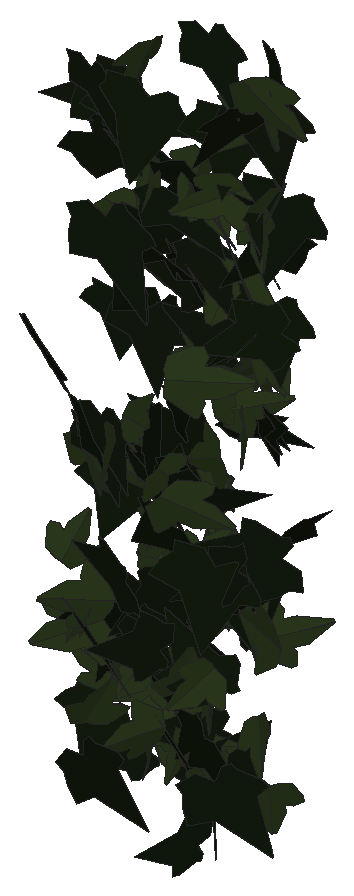
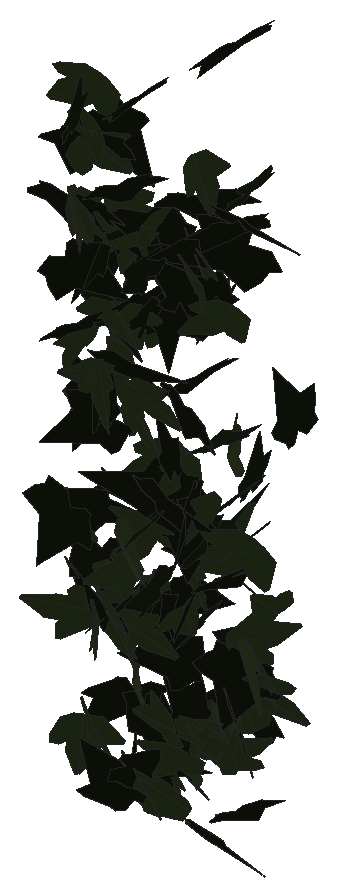
# SketchUp Ruby script. Lengths in inches.
U = 1.inch
M = Sketchup.active_model
def pt(a) = Geom::Point3d.new(a.map { |v| v * U })
def face(e, loops, mat)
  f = e.add_face(loops[0].map { |a| pt(a) })
  loops[1..].each { |l| e.add_face(l.map { |a| pt(a) }).erase! }
  f.material = f.back_material = mat if mat
  f
end
# faces: each face lists its corners as indices into pts; further lists are holes
def faces(e, pts, list, mat = nil) = list.each { |f| face(e, (f[0].is_a?(Array) ? f : [f]).map { |l| l.map { |i| pts[i] } }, mat) }
# xy, xz, yz: faces in a plane at the given z, y or x. An outline is a flat list of corners, or four numbers for a rectangle; further outlines are holes
def ring(l) = l.size == 4 ? [[l[0], l[1]], [l[2], l[1]], [l[2], l[3]], [l[0], l[3]]] : l.each_slice(2).to_a
def flat(e, list, mat, &to3) = list.each { |f| face(e, (f[0].is_a?(Array) ? f : [f]).map { |l| ring(l).map { |u, v| to3.(u, v) } }, mat) }
def xy(e, z, list, mat = nil) = flat(e, list, mat) { |x, y| [x, y, z] }
def xz(e, y, list, mat = nil) = flat(e, list, mat) { |x, z| [x, y, z] }
def yz(e, x, list, mat = nil) = flat(e, list, mat) { |y, z| [x, y, z] }
def lines(e, pts, list) = list.each { |a, b| e.add_line(pt(pts[a]), pt(pts[b])) }
# prism: a flat outline (further loops are holes) pulled along v
def prism(e, loops, v, mat = nil)
  f = face(e, loops, mat); d = Geom::Vector3d.new(v.map { |x| x * U })
  f.pushpull(f.normal.samedirection?(d) ? d.length : -d.length)
end
def box(e, o, s, mat = nil) = prism(e, [[o, [o[0] + s[0], o[1], o[2]], [o[0] + s[0], o[1] + s[1], o[2]], [o[0], o[1] + s[1], o[2]]]], [0, 0, s[2]], mat)
def at(x, y, z, deg = 0) = Geom::Transformation.translation(pt([x, y, z])) * Geom::Transformation.rotation(ORIGIN, Z_AXIS, deg.degrees)
def axes(o, x, y, z) = Geom::Transformation.new([*x, 0, *y, 0, *z, 0, *pt(o).to_a, 1])
def part(name) = M.definitions.add(name)
# library, detail: a bought-in or finely detailed component or shape, given as its bounding box
def library(name, o, s) = part(name).tap { |d| box(d.entities, o, s) }
def detail(e, o, s) = box(e.add_group.entities, o, s)
def put(e, d, t, mat = nil) = e.add_instance(d, t).tap { |i| i.material = mat if mat }
def group(e, t, mat = nil) = e.add_group.tap { |g| g.transformation = t; g.material = mat if mat }.entities
root = M.entities
M.materials.add("1026 AP 7946 SUNNY SIDE UP").color = [254, 231, 186]
M.materials.add("efeu1").color = [18, 25, 13]
M.materials.add("efeu2").color = [43, 57, 29]
c1 = part("ivyleaf_9")
p = [[1.54,2.16,1.25],[1.36,2.04,1.19],[-0.21,0.99,0.68],[-0.71,1.11,0.82],[-0.85,0.86,0.67],[-0.8,0.17,0.21],
  [-0.9,-0.01,0.1],[-0.67,-0.16,-0.02],[-0.08,-0.08,-0.05],[-0.03,-0.6,-0.4],[0.65,-0.88,-0.66],[0.83,-0.6,-0.49],
  [1.29,-0.42,-0.43],[1.8125,-0.07,-0.26],[1.21,0.44,0.15]]
faces(c1.entities,p,[[0,1,2,3,4,5,6,7,8,9,10,11,12,13,14]],"efeu1")
c2 = part("ivyleaf_10")
p = [[0,0.5,-0.03],[-0.0625,2.02,-0.43],[-0.19,2.01,-0.46],[-0.54,1.05,-0.29],[-0.52,0.625,-0.18],[-0.83,0.76,-0.28],
  [-1.16,0.64,-0.33],[-1.15,0.33,-0.24],[-0.77,-0.39,0.02],[-0.3,-0.51,0.16],[0.04,-0.48,0.23],[-0.02,2.01,-0.4375],
  [-0.06,2.01,-0.43],[0.04,-0.49,0.23],[0.67,-0.49,0.14],[1.38,0.36,-0.2],[1.375,0.51,-0.24],[0.81,0.65,-0.19],
  [0.62,0.59,-0.15],[0.6,1.09,-0.28],[0.5,1.23,-0.31]]
faces(c2.entities,p,[[0,1,2,3,4,5,6,7,8,9,10],[11,12,0,13,14,15,16,17,18,19,20]],"efeu2")
put(root,c1,axes([127.27,207.86,278.51],[0.09991,-0.42403,-0.09348],[-0.00995,0.08836,-0.44114],[0.68098,0.0635,0.00727]),"1026 AP 7946 SUNNY SIDE UP")
put(root,c1,axes([126.99,209.29,271.18],[-0.37733,0.18301,0.11018],[-0.15539,0.04456,-0.30973],[-0.29394,-0.25849,0.0223]),"1026 AP 7946 SUNNY SIDE UP")
put(root,c1,axes([125.64,209.45,268.95],[-0.00188,-0.09667,-0.35246],[0.53425,0.09867,-0.02942],[0.16176,-0.32702,0.09306]),"1026 AP 7946 SUNNY SIDE UP")
put(root,c1,axes([125.98,209.8125,271.66],[0.16936,-0.34122,-0.00918],[0.03095,-0.00109,0.36812],[-0.53575,-0.10793,0.01836]),"1026 AP 7946 SUNNY SIDE UP")
put(root,c1,axes([127.4,210,272.25],[-0.29374,-0.33207,-0.04474],[0.06069,0.02588,-0.39177],[0.5227,-0.18962,0.02034]),"1026 AP 7946 SUNNY SIDE UP")
put(root,c1,axes([127.26,209.77,268.05],[-0.34107,0.22543,0.04372],[-0.06924,0.01462,-0.32145],[-0.35361,-0.2203,0.02077]),"1026 AP 7946 SUNNY SIDE UP")
put(root,c2,axes([125.53,210.08,273.42],[0.03461,-0.00665,0.3661],[0.31545,-0.29372,-0.02018],[0.46141,0.20131,-0.01366]),"1026 AP 7946 SUNNY SIDE UP")
put(root,c2,axes([127.24,210.04,270.52],[0.16585,0.14434,-0.27042],[-0.20229,-0.23045,-0.18458],[-0.42663,0.16538,-0.01761]),"1026 AP 7946 SUNNY SIDE UP")
put(root,c2,axes([126.84,210.03,270.27],[-0.20114,-0.2859,-0.02326],[-0.0199,-0.01729,0.32254],[-0.45032,0.12847,-0.00387]),"1026 AP 7946 SUNNY SIDE UP")
put(root,c1,axes([125.02,210.1875,270.45],[0.25152,-0.2589,0.1894],[0.11164,-0.17317,-0.31337],[0.48804,0.17304,-0.02593]),"1026 AP 7946 SUNNY SIDE UP")
put(root,c1,axes([124.21,210.29,274.39],[0.02602,-0.13736,0.34062],[0.15547,-0.31717,-0.14236],[0.54225,0.09753,0.02447]),"1026 AP 7946 SUNNY SIDE UP")
put(root,c1,axes([126.1,210.04,270.95],[0.15449,-0.22762,-0.19575],[-0.12607,0.17091,-0.25436],[0.44751,0.12673,-0.00408]),"1026 AP 7946 SUNNY SIDE UP")
put(root,c2,axes([126.93,209.9,275.06],[0.05772,-0.07931,-0.37891],[0.47007,0.22983,-0.019],[0.3581,-0.28892,0.08601]),"1026 AP 7946 SUNNY SIDE UP")
put(root,c1,axes([127.65,210.14,272.23],[-0.43689,0.15575,-0.01515],[0.00086,-0.03079,-0.32718],[-0.24612,-0.27657,0.02575]),"1026 AP 7946 SUNNY SIDE UP")
put(root,c2,axes([125.21,210.12,269.19],[-0.17822,-0.27692,0.07402],[0.03531,0.07013,0.30861],[-0.4491,0.11541,-0.00511]),"1026 AP 7946 SUNNY SIDE UP")
put(root,c1,axes([127.4,210.08,268.9],[-0.01795,-0.22714,-0.28826],[0.05185,0.27683,-0.23235],[0.56274,-0.03275,0.01221]),"1026 AP 7946 SUNNY SIDE UP")
put(root,c1,axes([126.53,210.125,272.57],[0.14554,0.01847,-0.30587],[-0.45919,-0.05415,-0.09754],[-0.08995,0.30634,0.00305]),"1026 AP 7946 SUNNY SIDE UP")
put(root,c1,axes([124.9,210.47,273.28],[-0.0612,-0.09787,0.31696],[-0.00972,-0.31016,-0.10408],[0.5084,-0.01771,0.03616]),"1026 AP 7946 SUNNY SIDE UP")
put(root,c1,axes([127.17,210.23,270.29],[-0.39411,-0.2107,0.0742],[0.06415,0.06497,0.33687],[-0.34482,0.2529,-0.02213]),"1026 AP 7946 SUNNY SIDE UP")
put(root,c2,axes([126.62,210.11,272.98],[-0.24055,-0.14641,-0.30892],[0.38349,0.17475,-0.21566],[0.3564,-0.28686,0.02355]),"1026 AP 7946 SUNNY SIDE UP")
put(root,c2,axes([124.96,210.54,270.7],[0.00384,0.10084,0.37452],[-0.09963,-0.3577,0.10072],[0.58391,-0.0617,0.01472]),"1026 AP 7946 SUNNY SIDE UP")
put(root,c2,axes([125.82,210.59,268.97],[0.00712,-0.02337,0.36221],[-0.00975,-0.3517,-0.02605],[0.55418,-0.00589,-0.00512]),"1026 AP 7946 SUNNY SIDE UP")
put(root,c1,axes([125.49,210.66,275.79],[-0.06401,-0.17767,0.34495],[-0.0686,-0.33335,-0.18907],[0.59349,-0.05769,0.01535]),"1026 AP 7946 SUNNY SIDE UP")
put(root,c1,axes([126.07,210.77,271.18],[-0.01476,-0.05724,-0.38375],[0.18924,-0.35322,0.05077],[-0.56104,-0.11764,0.02722]),"1026 AP 7946 SUNNY SIDE UP")
put(root,c2,axes([126.57,210.73,268.27],[-0.00143,-0.11934,0.32477],[0.28541,-0.26659,-0.10476],[0.44781,0.16953,0.06781]),"1026 AP 7946 SUNNY SIDE UP")
put(root,c2,axes([127.12,210.4,273.7],[-0.20162,0.12835,0.2681],[-0.40277,0.082,-0.17168],[-0.21219,-0.27761,0.07113]),"1026 AP 7946 SUNNY SIDE UP")
put(root,c2,axes([126.2,210.4,273.15],[-0.10446,-0.21988,-0.21946],[0.16823,0.18622,-0.23266],[0.44958,-0.12077,0.03607]),"1026 AP 7946 SUNNY SIDE UP")
put(root,c2,axes([124.68,210.57,270.49],[0.28346,-0.25845,-0.03715],[-0.04145,0.02377,-0.32438],[0.40792,0.18201,-0.00715]),"1026 AP 7946 SUNNY SIDE UP")
put(root,c2,axes([124.68,210.68,270.14],[0.36279,0.00726,-0.25397],[-0.38216,-0.05104,-0.23614],[-0.06633,0.3338,-0.02858]),"1026 AP 7946 SUNNY SIDE UP")
put(root,c1,axes([126.74,210.8,268.31],[-0.03358,-0.01568,-0.35261],[0.4759,-0.16144,-0.01278],[-0.25226,-0.30247,0.02283]),"1026 AP 7946 SUNNY SIDE UP")
put(root,c2,axes([127.26,210.37,274.67],[0.02198,0.06976,0.31894],[-0.10522,0.30317,-0.06557],[-0.48717,-0.06233,0.02855]),"1026 AP 7946 SUNNY SIDE UP")
put(root,c1,axes([127.9,210.72,275.73],[-0.46783,0.00402,0.10863],[-0.16563,-0.02873,-0.30531],[0.00915,-0.31434,0.02744]),"1026 AP 7946 SUNNY SIDE UP")
put(root,c2,axes([125.625,210.82,268.53],[-0.05408,0.05838,0.32312],[0.30635,-0.24555,0.06773],[0.3966,0.19763,-0.00826]),"1026 AP 7946 SUNNY SIDE UP")
put(root,c2,axes([124.5,210.43,271.34],[0.13703,0.18573,-0.23167],[0.12732,0.21121,0.21229],[0.44192,-0.11845,0.01068]),"1026 AP 7946 SUNNY SIDE UP")
put(root,c1,axes([126.02,210.88,268.625],[-0.07889,-0.08642,0.34051],[0.11879,-0.3291,-0.07864],[0.52467,0.06152,0.06901]),"1026 AP 7946 SUNNY SIDE UP")
put(root,c1,axes([126.95,210.9,276.65],[0.2821,-0.17295,-0.30518],[0.44193,-0.11567,0.24506],[-0.30689,-0.32555,0.07237]),"1026 AP 7946 SUNNY SIDE UP")
put(root,c2,axes([127.98,210.45,271.16],[0.04232,-0.07884,-0.38868],[-0.34476,0.30738,-0.08058],[0.49762,0.21966,-0.02277]),"1026 AP 7946 SUNNY SIDE UP")
put(root,c2,axes([124.93,210.51,272.82],[-0.14254,0.25438,0.15434],[-0.09747,0.13528,-0.27717],[-0.45268,-0.10923,0.01108]),"1026 AP 7946 SUNNY SIDE UP")
put(root,c1,axes([124.81,210.83,273.3],[0.10859,-0.32056,0.01121],[-0.00415,-0.01356,-0.33785],[0.50442,0.06889,-0.00519]),"1026 AP 7946 SUNNY SIDE UP")
put(root,c1,axes([127.79,210.87,272.17],[-0.14084,-0.14988,-0.31774],[-0.32064,-0.23192,0.17624],[-0.432,0.22099,-0.02722]),"1026 AP 7946 SUNNY SIDE UP")
put(root,c1,axes([126.26,210.5625,272.63],[0.14978,0.04082,0.33982],[0.51087,0.05978,-0.104],[-0.10848,0.33787,-0.02059]),"1026 AP 7946 SUNNY SIDE UP")
put(root,c1,axes([126.69,210.65,269.11],[0.20222,-0.02875,-0.33271],[-0.50958,-0.01195,-0.13199],[-0.0008,0.34727,-0.03004]),"1026 AP 7946 SUNNY SIDE UP")
put(root,c1,axes([127.47,210.74,275.58],[-0.26572,0.25247,-0.09249],[0.06154,-0.08346,-0.31317],[-0.41759,-0.17295,0.0127]),"1026 AP 7946 SUNNY SIDE UP")
put(root,c2,axes([126.55,210.99,269.73],[0.11557,-0.11452,0.32943],[0.32122,-0.24731,-0.14078],[0.4279,0.21659,0.01671]),"1026 AP 7946 SUNNY SIDE UP")
put(root,c2,axes([126.67,210.55,271.79],[0.14921,0.14974,-0.31156],[0.18275,0.28137,0.18223],[0.49945,-0.14769,0.0264]),"1026 AP 7946 SUNNY SIDE UP")
put(root,c2,axes([127.14,211.03,274.13],[0.15521,-0.20932,0.29815],[0.28379,-0.23129,-0.23614],[0.48641,0.20174,0.04263]),"1026 AP 7946 SUNNY SIDE UP")
put(root,c1,axes([125.51,210.82,270.98],[0.26552,-0.27145,-0.12209],[-0.08652,0.10349,-0.32865],[0.45665,0.17744,0.00872]),"1026 AP 7946 SUNNY SIDE UP")
put(root,c1,axes([125.39,210.94,275.99],[0.1155,-0.09534,0.29048],[0.28402,-0.21726,-0.12519],[0.37301,0.19495,0.00538]),"1026 AP 7946 SUNNY SIDE UP")
put(root,c1,axes([124.83,210.68,270.42],[0.33032,0.24724,-0.03375],[-0.01325,-0.0376,-0.33395],[-0.39224,0.20948,-0.01714]),"1026 AP 7946 SUNNY SIDE UP")
put(root,c1,axes([125.45,211.03,275.09],[-0.03538,-0.37488,0.0251],[0.00109,-0.02658,-0.38704],[0.59093,-0.02239,0.00222]),"1026 AP 7946 SUNNY SIDE UP")
put(root,c2,axes([127.67,210.84,268.53],[-0.33662,-0.25238,-0.03652],[0.05863,0.0129,-0.34024],[0.39612,-0.21638,0.01932]),"1026 AP 7946 SUNNY SIDE UP")
put(root,c1,axes([125.51,211.04,269.52],[0.05115,-0.0848,0.32343],[0.19244,-0.28965,-0.09521],[0.47454,0.1266,0.00375]),"1026 AP 7946 SUNNY SIDE UP")
put(root,c2,axes([127.26,210.65,274.41],[0.04171,-0.0045,-0.34676],[0.34711,0.2551,0.0159],[0.39954,-0.22115,0.02238]),"1026 AP 7946 SUNNY SIDE UP")
put(root,c1,axes([124.47,211.03,278.45],[0.11901,-0.30664,0.06791],[0.03001,-0.06498,-0.32574],[0.49284,0.078,0.00344]),"1026 AP 7946 SUNNY SIDE UP")
put(root,c2,axes([125.86,210.86,271.97],[0.35971,-0.22556,-0.15011],[-0.16316,0.10047,-0.33037],[0.38825,0.2512,0.00023]),"1026 AP 7946 SUNNY SIDE UP")
put(root,c2,axes([126.85,211.05,277.375],[0.22311,0.08163,-0.30419],[-0.38043,-0.17057,-0.16909],[-0.29662,0.28017,-0.01193]),"1026 AP 7946 SUNNY SIDE UP")
put(root,c1,axes([127.32,210.81,271.49],[-0.0268,0.34631,-0.09795],[-0.00633,-0.09734,-0.35766],[-0.56548,-0.01532,0.00864]),"1026 AP 7946 SUNNY SIDE UP")
put(root,c1,axes([127.07,210.97,278.6875],[-0.06803,0.25081,-0.24763],[0.06298,-0.23846,-0.2636],[-0.54418,-0.05896,0.00045]),"1026 AP 7946 SUNNY SIDE UP")
put(root,c2,axes([127.36,210.96,279.17],[-0.3807,-0.00009,-0.24392],[0.36636,-0.06033,-0.24578],[-0.06622,-0.33323,0.04255]),"1026 AP 7946 SUNNY SIDE UP")
put(root,c1,axes([126.39,210.86,270.77],[0.10181,-0.09867,0.27903],[-0.1404,0.25768,0.11995],[-0.43185,-0.10704,0.02678]),"1026 AP 7946 SUNNY SIDE UP")
put(root,c2,axes([125.99,211.04,268.63],[0.32056,-0.20487,0.05146],[0.03358,-0.05068,-0.29731],[0.33031,0.20397,-0.01971]),"1026 AP 7946 SUNNY SIDE UP")
put(root,c2,axes([127.04,210.73,274.58],[0.06583,-0.04009,0.32051],[-0.05262,0.31174,0.04781],[-0.49078,-0.0388,0.03787]),"1026 AP 7946 SUNNY SIDE UP")
put(root,c1,axes([126.26,211.2,275.73],[-0.09104,0.0095,0.33014],[-0.34085,-0.24102,-0.0344],[0.37132,-0.21892,0.04937]),"1026 AP 7946 SUNNY SIDE UP")
put(root,c1,axes([125.42,210.92,276.26],[-0.10622,-0.03832,0.30642],[0.47125,0.00731,0.07108],[-0.02463,0.30513,0.03859]),"1026 AP 7946 SUNNY SIDE UP")
put(root,c2,axes([127.21,211.15,277.03],[0.31563,-0.09633,0.22963],[0.2801,-0.13914,-0.22747],[0.26063,0.26619,-0.03361]),"1026 AP 7946 SUNNY SIDE UP")
put(root,c1,axes([127.09,211.21,274.01],[-0.00037,-0.07222,0.35978],[0.21834,-0.32214,-0.07034],[0.5172,0.13594,0.02995]),"1026 AP 7946 SUNNY SIDE UP")
put(root,c2,axes([125.36,211.13,277.23],[0.35508,-0.17658,0.11695],[0.11653,-0.09051,-0.29482],[0.30974,0.23647,-0.02316]),"1026 AP 7946 SUNNY SIDE UP")
put(root,c1,axes([125.77,211.18,273.59],[-0.01857,0.03451,0.30122],[0.08363,-0.28736,0.0355],[0.45502,0.05422,0.00577]),"1026 AP 7946 SUNNY SIDE UP")
put(root,c2,axes([124.57,211.01,270.83],[0.1814,-0.33764,-0.12243],[-0.08,0.10609,-0.3667],[0.55611,0.1254,-0.01282]),"1026 AP 7946 SUNNY SIDE UP")
put(root,c1,axes([125.25,211.23,278.19],[-0.31977,-0.3193,-0.04958],[0.06651,0.02789,-0.38925],[0.50294,-0.2067,0.01995]),"1026 AP 7946 SUNNY SIDE UP")
put(root,c1,axes([124.45,211.2,272.82],[0.07282,-0.32278,0.02636],[-0.00106,-0.0278,-0.33606],[0.50937,0.04608,-0.00447]),"1026 AP 7946 SUNNY SIDE UP")
put(root,c1,axes([125.875,211.08,277.17],[0.19198,-0.05348,0.29158],[0.41463,-0.10377,-0.13785],[0.18343,0.29055,0.00641]),"1026 AP 7946 SUNNY SIDE UP")
put(root,c2,axes([124.8125,211.15,269.19],[0.20131,0.17687,0.21535],[-0.23465,-0.1471,0.22258],[0.35957,-0.19501,0.02469]),"1026 AP 7946 SUNNY SIDE UP")
put(root,c2,axes([126.07,211.32,277.42],[-0.10076,-0.16907,0.29259],[0.18064,-0.28358,-0.14837],[0.4887,0.06996,0.11517]),"1026 AP 7946 SUNNY SIDE UP")
put(root,c1,axes([125.16,211.2,272.62],[0.28068,-0.2741,0.0578],[0.02707,-0.05751,-0.33687],[0.43959,0.17855,-0.01616]),"1026 AP 7946 SUNNY SIDE UP")
put(root,c1,axes([125.5,211.13,270.48],[0.36752,-0.10729,0.17138],[0.22062,-0.09312,-0.26453],[0.22072,0.27173,-0.02096]),"1026 AP 7946 SUNNY SIDE UP")
put(root,c2,axes([124.91,211.17,269.72],[0.2424,-0.2602,0.03119],[0.00742,-0.03408,-0.31147],[0.4121,0.15366,-0.01274]),"1026 AP 7946 SUNNY SIDE UP")
put(root,c1,axes([124.78,211.32,272.14],[-0.18928,-0.27841,0.08752],[-0.02363,-0.08757,-0.3123],[0.45783,-0.11962,0.02006]),"1026 AP 7946 SUNNY SIDE UP")
put(root,c1,axes([127.28,211.05,274.15],[0.40055,-0.05505,-0.15228],[-0.23815,-0.00906,-0.26603],[0.06762,0.29422,-0.0349]),"1026 AP 7946 SUNNY SIDE UP")
put(root,c2,axes([125.54,211.2,271.34],[0.14194,0.29236,-0.1596],[-0.05313,-0.15333,-0.31589],[-0.51878,0.09569,-0.01131]),"1026 AP 7946 SUNNY SIDE UP")
put(root,c1,axes([124.88,210.94,269.86],[-0.07016,-0.02666,-0.35582],[-0.5006,0.14006,0.03207],[0.21413,0.31869,-0.04162]),"1026 AP 7946 SUNNY SIDE UP")
put(root,c1,axes([126,211.2,271.51],[0.27746,-0.26206,-0.00956],[-0.03093,-0.00387,-0.32493],[0.41108,0.17658,-0.018]),"1026 AP 7946 SUNNY SIDE UP")
put(root,c2,axes([125.34,211.17,269.41],[0.40659,-0.09143,-0.13996],[-0.2176,0.01195,-0.28063],[0.1364,0.29161,-0.0305]),"1026 AP 7946 SUNNY SIDE UP")
put(root,c1,axes([124.43,211.34,268.52],[-0.20245,-0.26902,0.06509],[-0.01618,-0.06667,-0.30701],[0.43478,-0.12775,0.01888]),"1026 AP 7946 SUNNY SIDE UP")
put(root,c1,axes([125.98,211.02,276.06],[0.27189,0.01759,-0.26305],[-0.40133,0.03637,-0.1752],[0.03204,0.30631,0.03773]),"1026 AP 7946 SUNNY SIDE UP")
put(root,c1,axes([127.54,211.29,277.39],[-0.47332,-0.16198,-0.17758],[0.2614,0.0515,-0.3505],[0.2631,-0.34257,0.02878]),"1026 AP 7946 SUNNY SIDE UP")
put(root,c2,axes([125.18,211.2,269.55],[0.46399,0.01283,-0.08631],[-0.12952,-0.0292,-0.30339],[-0.03188,0.30537,-0.02358]),"1026 AP 7946 SUNNY SIDE UP")
put(root,c1,axes([125.79,211.13,276.98],[-0.07578,-0.17867,-0.25963],[0.20206,0.21925,-0.18491],[0.44031,-0.13137,0.04017]),"1026 AP 7946 SUNNY SIDE UP")
put(root,c1,axes([126.25,211.2,276.22],[0.06096,-0.28527,-0.12488],[-0.01328,0.11951,-0.2958],[0.4862,0.03903,0.00758]),"1026 AP 7946 SUNNY SIDE UP")
put(root,c1,axes([124.6,211,277.52],[0.05538,0.01723,-0.38565],[0.30228,0.32203,0.03578],[0.50598,-0.19427,0.02083]),"1026 AP 7946 SUNNY SIDE UP")
put(root,c2,axes([126.17,211.2,267.95],[0.39184,-0.2261,-0.13134],[0.17529,-0.06442,0.34527],[-0.3675,-0.27181,0.02464]),"1026 AP 7946 SUNNY SIDE UP")
put(root,c2,axes([126.83,211.04,271.25],[0.07454,-0.22604,0.21101],[-0.04456,0.20442,0.23888],[-0.47893,-0.0542,0.01061]),"1026 AP 7946 SUNNY SIDE UP")
put(root,c2,axes([127.44,211.08,275.11],[0.04212,0.30212,0.09354],[0.01983,0.0883,-0.31191],[-0.49488,0.02925,-0.00454]),"1026 AP 7946 SUNNY SIDE UP")
put(root,c1,axes([126.29,211.29,279.48],[0.08982,-0.3422,-0.05207],[-0.01132,0.04808,-0.35713],[0.54337,0.05757,0.00117]),"1026 AP 7946 SUNNY SIDE UP")
put(root,c1,axes([126.6,211.24,271.14],[0.20801,-0.30872,-0.08606],[-0.06128,0.07226,-0.34551],[0.49843,0.13773,-0.00656]),"1026 AP 7946 SUNNY SIDE UP")
put(root,c2,axes([126.36,211.24,274.61],[-0.28339,0.02414,0.24134],[-0.35295,-0.10634,-0.16733],[0.11134,-0.27566,0.08382]),"1026 AP 7946 SUNNY SIDE UP")
put(root,c2,axes([124.4,211.18,272.68],[-0.39778,-0.04313,-0.27453],[0.42334,-0.01858,-0.26055],[0.02534,-0.36679,0.0433]),"1026 AP 7946 SUNNY SIDE UP")
put(root,c1,axes([125.5,211.14,272.78],[0.33868,0.10817,-0.17075],[-0.22596,-0.08429,-0.24863],[-0.21518,0.25877,-0.00767]),"1026 AP 7946 SUNNY SIDE UP")
put(root,c1,axes([126.98,211.08,273.89],[0.3787,0.10963,0.14266],[0.2027,0.04941,-0.27221],[-0.18871,0.27307,-0.00611]),"1026 AP 7946 SUNNY SIDE UP")
put(root,c1,axes([124.83,211.29,278.1],[-0.40716,0.10952,0.1369],[-0.22915,-0.01355,-0.28243],[-0.14284,-0.29045,0.06286]),"1026 AP 7946 SUNNY SIDE UP")
put(root,c2,axes([124.78,211.19,276.41],[-0.24805,-0.14262,-0.22732],[0.36085,0.04871,-0.20191],[0.19894,-0.26617,0.0828]),"1026 AP 7946 SUNNY SIDE UP")
put(root,c1,axes([126.73,211.22,274.9],[-0.14319,0.13785,0.25608],[-0.4012,0.07368,-0.1384],[-0.19448,-0.2535,0.09697]),"1026 AP 7946 SUNNY SIDE UP")
put(root,c2,axes([126.09,211.29,272.55],[0.4304,0.06531,0.13793],[0.21643,-0.00577,-0.28782],[-0.08821,0.3045,-0.03317]),"1026 AP 7946 SUNNY SIDE UP")
put(root,c2,axes([127.05,211.47,278.47],[-0.26628,-0.13594,0.26767],[-0.11402,-0.27214,-0.19638],[0.44788,-0.1501,0.10915]),"1026 AP 7946 SUNNY SIDE UP")
put(root,c1,axes([125.42,211.11,273.22],[0.17125,-0.12531,-0.34395],[-0.4013,0.21536,-0.16814],[0.39013,0.27653,-0.02198]),"1026 AP 7946 SUNNY SIDE UP")
put(root,c1,axes([126.86,211.25,270.64],[-0.20475,0.20253,0.25421],[0.21581,-0.20371,0.24683],[0.45165,0.18915,-0.0027]),"1026 AP 7946 SUNNY SIDE UP")
put(root,c2,axes([126.62,211.34,275.92],[0.52936,0.09122,-0.07121],[-0.09114,-0.05116,-0.35796],[-0.15576,0.33995,-0.03259]),"1026 AP 7946 SUNNY SIDE UP")
put(root,c1,axes([124.55,211.37,278.03],[-0.03835,-0.3407,-0.12939],[0.0464,0.12167,-0.3506],[0.56802,-0.03294,0.0199]),"1026 AP 7946 SUNNY SIDE UP")
put(root,c2,axes([126.25,211.21,277.12],[0.15751,0.27947,0.09608],[0.07385,0.08041,-0.30491],[-0.45654,0.10943,-0.01618]),"1026 AP 7946 SUNNY SIDE UP")
put(root,c2,axes([127.34,211.38,277.375],[0.02148,-0.31131,0.06987],[0.02624,-0.06886,-0.32112],[0.5009,0.01695,0.01383]),"1026 AP 7946 SUNNY SIDE UP")
put(root,c2,axes([126.97,211.45,269.02],[0.29492,-0.11989,0.22527],[0.26537,-0.14156,-0.22921],[0.28995,0.2515,-0.01935]),"1026 AP 7946 SUNNY SIDE UP")
put(root,c1,axes([127.01,211.25,276.77],[0.36441,-0.1361,-0.18069],[-0.25833,0.06374,-0.27542],[0.23336,0.28309,-0.02273]),"1026 AP 7946 SUNNY SIDE UP")
put(root,c2,axes([126.65,211.08,271.63],[-0.02199,-0.04926,-0.34803],[0.23354,0.30325,-0.05015],[0.48287,-0.14891,0.0084]),"1026 AP 7946 SUNNY SIDE UP")
put(root,c1,axes([125.97,211.51,276.78],[0.13261,-0.20306,0.22921],[0.14263,-0.20445,-0.22768],[0.45306,0.1238,0.00459]),"1026 AP 7946 SUNNY SIDE UP")
put(root,c1,axes([126.24,211.54,268.6875],[-0.07521,-0.14969,-0.27574],[-0.10614,-0.25823,0.16021],[-0.46919,0.08241,0.00796]),"1026 AP 7946 SUNNY SIDE UP")
put(root,c2,axes([125.55,211.29,268.98],[0.32516,0.15442,0.17423],[0.24304,0.07244,-0.26379],[-0.26434,0.25656,-0.02822]),"1026 AP 7946 SUNNY SIDE UP")
put(root,c2,axes([124.72,211.27,269.32],[-0.26778,0.28029,-0.08297],[-0.06187,0.07219,0.33827],[0.45507,0.17474,-0.00283]),"1026 AP 7946 SUNNY SIDE UP")
put(root,c1,axes([126.45,211.53,278.08],[-0.17721,-0.31765,0.00216],[0.01554,-0.00765,-0.34706],[0.49927,-0.11251,0.01157]),"1026 AP 7946 SUNNY SIDE UP")
put(root,c2,axes([126.83,211.4,271.15],[0.32525,-0.24644,-0.02255],[-0.04431,0.00305,-0.33083],[0.38631,0.20784,-0.01896]),"1026 AP 7946 SUNNY SIDE UP")
put(root,c1,axes([127.21,211.52,275.5625],[-0.0857,-0.34786,-0.01326],[0.01821,0.00921,-0.36253],[0.54694,-0.05481,0.00999]),"1026 AP 7946 SUNNY SIDE UP")
put(root,c2,axes([127.2,211.13,270.59],[-0.05398,0.08042,0.34871],[-0.33792,0.262,-0.08516],[-0.42932,-0.21633,0.02319]),"1026 AP 7946 SUNNY SIDE UP")
put(root,c1,axes([126,211.64,272.6],[-0.03265,-0.29241,0.21526],[-0.02272,-0.21012,-0.30322],[0.56618,-0.02529,0.00025]),"1026 AP 7946 SUNNY SIDE UP")
put(root,c2,axes([126.37,211.46,270.9],[-0.21886,-0.05618,0.27084],[-0.3356,-0.15751,-0.15182],[0.25785,-0.25269,0.0323]),"1026 AP 7946 SUNNY SIDE UP")
put(root,c2,axes([125.04,211.55,277],[-0.21019,0.05226,-0.27876],[0.17106,-0.26663,-0.10986],[-0.39864,-0.14197,0.09984]),"1026 AP 7946 SUNNY SIDE UP")
put(root,c2,axes([127.02,211.45,278.74],[-0.33117,0.15875,-0.1756],[0.15016,-0.15204,-0.26692],[-0.3352,-0.22495,0.05391]),"1026 AP 7946 SUNNY SIDE UP")
put(root,c1,axes([125.33,211.58,271.25],[-0.07914,0.03878,0.30996],[-0.16216,-0.28878,0.0189],[0.44823,-0.09763,0.06156]),"1026 AP 7946 SUNNY SIDE UP")
put(root,c1,axes([127.11,211.46,278.6],[-0.2575,-0.23419,-0.18724],[0.18073,0.13959,-0.29332],[0.42828,-0.19971,0.0112]),"1026 AP 7946 SUNNY SIDE UP")
put(root,c2,axes([127.37,211.18,270.69],[0.12845,0.04736,-0.36456],[0.42748,0.22748,0.09727],[0.36454,-0.28345,0.01439]),"1026 AP 7946 SUNNY SIDE UP")
put(root,c2,axes([125.07,211.45,278.82],[-0.05645,-0.33029,0.04031],[0.00016,-0.04125,-0.34248],[0.52334,-0.03562,0.00445]),"1026 AP 7946 SUNNY SIDE UP")
put(root,c2,axes([125.57,211.42,268.29],[0.22507,-0.11322,-0.32961],[0.50519,-0.06459,0.17159],[-0.16898,-0.34391,0.07399]),"1026 AP 7946 SUNNY SIDE UP")
put(root,c1,axes([124.5,211.625,274.6],[-0.11223,-0.27303,0.12115],[0.0883,-0.13266,-0.27928],[0.46001,-0.04115,0.08317]),"1026 AP 7946 SUNNY SIDE UP")
put(root,c2,axes([125.04,211.2,273.19],[-0.02305,0.19423,0.24528],[-0.06652,0.2337,-0.19865],[-0.47719,-0.04196,0.01584]),"1026 AP 7946 SUNNY SIDE UP")
put(root,c1,axes([125.26,211.53,274.88],[-0.32522,-0.00488,-0.28824],[0.43792,-0.0371,-0.21166],[-0.04238,-0.34593,0.02472]),"1026 AP 7946 SUNNY SIDE UP")
put(root,c1,axes([125.08,211.43,268.02],[-0.38837,0.10982,0.07986],[-0.12761,0.00584,-0.27708],[-0.1678,-0.25862,0.02587]),"1026 AP 7946 SUNNY SIDE UP")
put(root,c2,axes([126.49,211.47,270.79],[0.29321,-0.24823,-0.00718],[-0.02817,-0.00652,-0.31932],[0.38939,0.18644,-0.0177]),"1026 AP 7946 SUNNY SIDE UP")
put(root,c1,axes([127.33,211.58,276.6],[-0.04961,0.10077,-0.32324],[0.03591,-0.31435,-0.10802],[-0.5178,-0.03145,0.02348]),"1026 AP 7946 SUNNY SIDE UP")
put(root,c2,axes([127.04,211.3125,274.73],[-0.37986,0.18292,0.19314],[-0.28062,0.06984,-0.3084],[-0.29987,-0.29706,0.04393]),"1026 AP 7946 SUNNY SIDE UP")
put(root,c2,axes([127.4,211.39,277.44],[0.13877,-0.31025,-0.10293],[-0.01803,0.09867,-0.33135],[0.51136,0.08767,0.01625]),"1026 AP 7946 SUNNY SIDE UP")
put(root,c1,axes([126.37,211.33,268.05],[-0.29907,-0.01653,0.32677],[0.49945,-0.00122,0.19608],[-0.01171,0.36993,0.01742]),"1026 AP 7946 SUNNY SIDE UP")
put(root,c2,axes([125.52,211.57,269.6],[0.13836,0.0163,0.31944],[0.47305,-0.08385,-0.08393],[0.12025,0.31113,-0.03739]),"1026 AP 7946 SUNNY SIDE UP")
put(root,c2,axes([126.28,211.62,272.36],[0.26204,-0.31779,0.11835],[0.05778,-0.11231,-0.36982],[0.52916,0.16963,-0.01823]),"1026 AP 7946 SUNNY SIDE UP")
put(root,c1,axes([125.88,211.35,273.02],[-0.12986,0.12382,0.30087],[-0.30733,0.21692,-0.15078],[-0.39158,-0.21132,0.01856]),"1026 AP 7946 SUNNY SIDE UP")
put(root,c1,axes([127.14,211.76,278.91],[-0.04862,-0.08207,0.32795],[-0.03832,-0.31876,-0.08884],[0.51622,-0.03139,0.0243]),"1026 AP 7946 SUNNY SIDE UP")
put(root,c1,axes([127.61,211.24,272.28],[0.16317,0.2997,0.16992],[0.10349,0.14984,-0.32564],[-0.52655,0.12233,-0.01135]),"1026 AP 7946 SUNNY SIDE UP")
